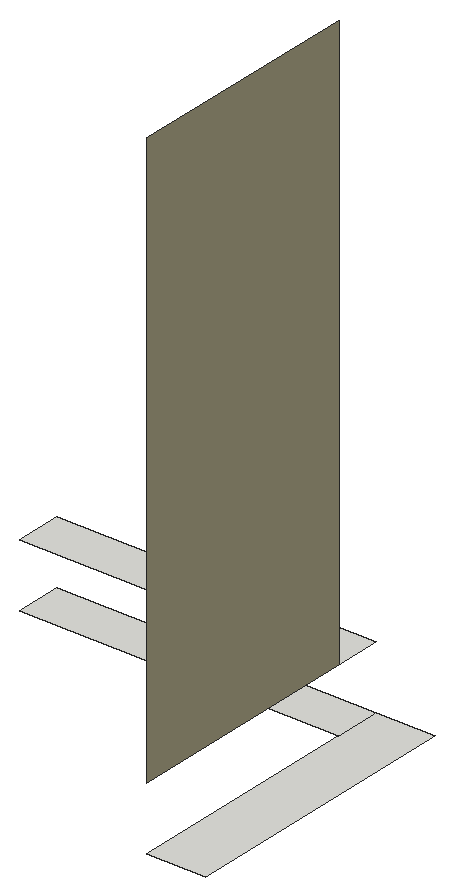
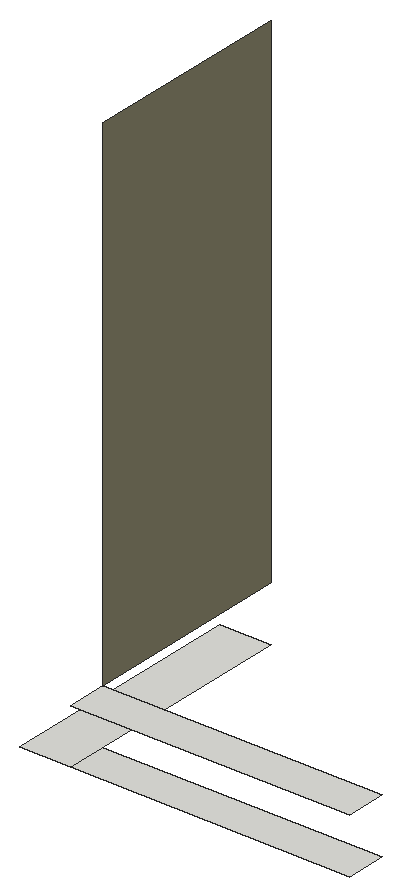
# SketchUp Ruby script. Lengths in inches.
U = 1.inch
M = Sketchup.active_model
def pt(a) = Geom::Point3d.new(a.map { |v| v * U })
def face(e, loops, mat)
  f = e.add_face(loops[0].map { |a| pt(a) })
  loops[1..].each { |l| e.add_face(l.map { |a| pt(a) }).erase! }
  f.material = f.back_material = mat if mat
  f
end
# faces: each face lists its corners as indices into pts; further lists are holes
def faces(e, pts, list, mat = nil) = list.each { |f| face(e, (f[0].is_a?(Array) ? f : [f]).map { |l| l.map { |i| pts[i] } }, mat) }
# xy, xz, yz: faces in a plane at the given z, y or x. An outline is a flat list of corners, or four numbers for a rectangle; further outlines are holes
def ring(l) = l.size == 4 ? [[l[0], l[1]], [l[2], l[1]], [l[2], l[3]], [l[0], l[3]]] : l.each_slice(2).to_a
def flat(e, list, mat, &to3) = list.each { |f| face(e, (f[0].is_a?(Array) ? f : [f]).map { |l| ring(l).map { |u, v| to3.(u, v) } }, mat) }
def xy(e, z, list, mat = nil) = flat(e, list, mat) { |x, y| [x, y, z] }
def xz(e, y, list, mat = nil) = flat(e, list, mat) { |x, z| [x, y, z] }
def yz(e, x, list, mat = nil) = flat(e, list, mat) { |y, z| [x, y, z] }
def lines(e, pts, list) = list.each { |a, b| e.add_line(pt(pts[a]), pt(pts[b])) }
# prism: a flat outline (further loops are holes) pulled along v
def prism(e, loops, v, mat = nil)
  f = face(e, loops, mat); d = Geom::Vector3d.new(v.map { |x| x * U })
  f.pushpull(f.normal.samedirection?(d) ? d.length : -d.length)
end
def box(e, o, s, mat = nil) = prism(e, [[o, [o[0] + s[0], o[1], o[2]], [o[0] + s[0], o[1] + s[1], o[2]], [o[0], o[1] + s[1], o[2]]]], [0, 0, s[2]], mat)
def at(x, y, z, deg = 0) = Geom::Transformation.translation(pt([x, y, z])) * Geom::Transformation.rotation(ORIGIN, Z_AXIS, deg.degrees)
def axes(o, x, y, z) = Geom::Transformation.new([*x, 0, *y, 0, *z, 0, *pt(o).to_a, 1])
def part(name) = M.definitions.add(name)
# library, detail: a bought-in or finely detailed component or shape, given as its bounding box
def library(name, o, s) = part(name).tap { |d| box(d.entities, o, s) }
def detail(e, o, s) = box(e.add_group.entities, o, s)
def put(e, d, t, mat = nil) = e.add_instance(d, t).tap { |i| i.material = mat if mat }
def group(e, t, mat = nil) = e.add_group.tap { |g| g.transformation = t; g.material = mat if mat }.entities
root = M.entities
M.materials.add("[Stone Coursed Rough]").color = [155, 150, 122]
xy(root,95.36,[[186.24,203.17,189.49,219.06],[168.55,216.5,186.24,219.06]])
xy(root,98.875,[[168.55,216.5,186.24,219.06]])
yz(root,186.24,[[203.17,98.875,216.5,130.875]],"[Stone Coursed Rough]")
